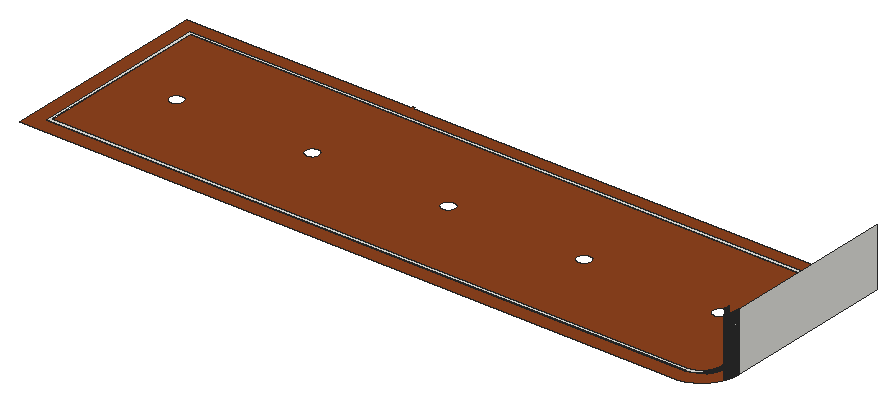
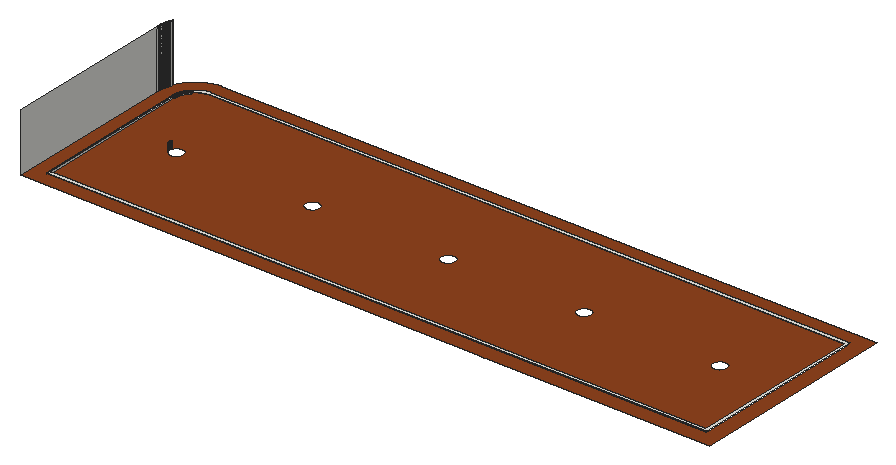
# SketchUp Ruby script. Lengths in inches.
U = 1.inch
M = Sketchup.active_model
def pt(a) = Geom::Point3d.new(a.map { |v| v * U })
def face(e, loops, mat)
  f = e.add_face(loops[0].map { |a| pt(a) })
  loops[1..].each { |l| e.add_face(l.map { |a| pt(a) }).erase! }
  f.material = f.back_material = mat if mat
  f
end
# faces: each face lists its corners as indices into pts; further lists are holes
def faces(e, pts, list, mat = nil) = list.each { |f| face(e, (f[0].is_a?(Array) ? f : [f]).map { |l| l.map { |i| pts[i] } }, mat) }
# xy, xz, yz: faces in a plane at the given z, y or x. An outline is a flat list of corners, or four numbers for a rectangle; further outlines are holes
def ring(l) = l.size == 4 ? [[l[0], l[1]], [l[2], l[1]], [l[2], l[3]], [l[0], l[3]]] : l.each_slice(2).to_a
def flat(e, list, mat, &to3) = list.each { |f| face(e, (f[0].is_a?(Array) ? f : [f]).map { |l| ring(l).map { |u, v| to3.(u, v) } }, mat) }
def xy(e, z, list, mat = nil) = flat(e, list, mat) { |x, y| [x, y, z] }
def xz(e, y, list, mat = nil) = flat(e, list, mat) { |x, z| [x, y, z] }
def yz(e, x, list, mat = nil) = flat(e, list, mat) { |y, z| [x, y, z] }
def lines(e, pts, list) = list.each { |a, b| e.add_line(pt(pts[a]), pt(pts[b])) }
# prism: a flat outline (further loops are holes) pulled along v
def prism(e, loops, v, mat = nil)
  f = face(e, loops, mat); d = Geom::Vector3d.new(v.map { |x| x * U })
  f.pushpull(f.normal.samedirection?(d) ? d.length : -d.length)
end
def box(e, o, s, mat = nil) = prism(e, [[o, [o[0] + s[0], o[1], o[2]], [o[0] + s[0], o[1] + s[1], o[2]], [o[0], o[1] + s[1], o[2]]]], [0, 0, s[2]], mat)
def at(x, y, z, deg = 0) = Geom::Transformation.translation(pt([x, y, z])) * Geom::Transformation.rotation(ORIGIN, Z_AXIS, deg.degrees)
def axes(o, x, y, z) = Geom::Transformation.new([*x, 0, *y, 0, *z, 0, *pt(o).to_a, 1])
def part(name) = M.definitions.add(name)
# library, detail: a bought-in or finely detailed component or shape, given as its bounding box
def library(name, o, s) = part(name).tap { |d| box(d.entities, o, s) }
def detail(e, o, s) = box(e.add_group.entities, o, s)
def put(e, d, t, mat = nil) = e.add_instance(d, t).tap { |i| i.material = mat if mat }
def group(e, t, mat = nil) = e.add_group.tap { |g| g.transformation = t; g.material = mat if mat }.entities
root = M.entities
M.materials.add("[Wood Fence]").color = [142, 67, 30]
xy(root,228,[[[99,214,99,300,191.5,300,191.5,300.5,192.5,300.5,192.5,300,383,300,383,229.12,382.99,228.93,382.98,228.73,382.96,228.35,382.86,227.4,382.74,226.64,382.7,226.46,382.58,225.89,382.53,225.71,382.48,225.52,382.43,225.34,382.38,225.15,382.33,224.97,382.27,224.79,382.21,224.6,382.09,224.24,382.02,224.0625,381.95,223.88,381.88,223.71,381.74,223.35,381.66,223.18,381.58,223,381.42,222.66,381.33,222.48,381.24,222.3125,381.15,222.14,381.0625,221.98,380.97,221.81,380.87,221.64,380.78,221.48,380.68,221.31,380.57,221.15,380.47,220.99,380.36,220.83,380.26,220.67,380.15,220.52,380.04,220.36,379.92,220.21,379.81,220.05,379.45,219.6,379.33,219.46,379.2,219.31,379.08,219.17,378.95,219.02,378.82,218.88,378.6875,218.74,378.56,218.61,378.15,218.2,378.01,218.07,377.86,217.94,377.72,217.8125,377.58,217.6875,377.43,217.56,376.98,217.2,376.83,217.09,376.68,216.97,376.52,216.86,376.37,216.75,376.05,216.53,375.89,216.43,375.73,216.32,375.57,216.22,375.4,216.125,375.24,216.03,375.07,215.93,374.91,215.84,374.4,215.57,374.22,215.49,374.05,215.41,373.88,215.32,373.7,215.25,373.53,215.17,373.35,215.1,373.17,215.02,372.99,214.95,372.82,214.89,372.64,214.82,372.45,214.76,371.91,214.58,371.72,214.53,371.54,214.48,371.35,214.43,371.17,214.38,370.98,214.34,370.8,214.29,370.61,214.25,370.42,214.22,370.23,214.18,369.85,214.12,369.67,214.09,369.48,214.0625,369.29,214.04,369.1,214.01,368.95,214],[105,220,368.62,220,368.6875,220.01,368.8,220.02,368.92,220.04,369.03,220.0625,369.15,220.08,369.27,220.1,369.38,220.13,369.5,220.15,369.61,220.18,369.73,220.21,369.84,220.23,369.95,220.27,370.07,220.3,370.29,220.36,370.41,220.4,370.52,220.4375,370.63,220.48,370.96,220.6,371.07,220.65,371.18,220.69,371.28,220.74,371.61,220.89,371.71,220.9375,371.82,220.99,371.92,221.05,372.02,221.1,372.23,221.22,372.63,221.46,372.73,221.53,372.83,221.59,372.92,221.66,373.02,221.73,373.11,221.8,373.21,221.87,373.39,222.01,373.49,222.09,373.58,222.16,373.76,222.32,373.84,222.39,374.02,222.55,374.1,222.64,374.18,222.72,374.27,222.8,374.35,222.89,374.43,222.97,374.67,223.24,374.74,223.32,374.82,223.42,374.89,223.51,374.97,223.6,375.04,223.69,375.11,223.79,375.18,223.88,375.25,223.98,375.3125,224.07,375.38,224.17,375.44,224.27,375.51,224.37,375.75,224.77,375.81,224.875,375.86,224.98,375.92,225.08,375.97,225.1875,376.03,225.29,376.08,225.4,376.125,225.51,376.18,225.61,376.22,225.72,376.27,225.83,376.3125,225.9375,376.36,226.05,376.4,226.16,376.4375,226.27,376.48,226.38,376.51,226.49,376.55,226.6,376.59,226.72,376.68,227.05,376.71,227.17,376.74,227.28,376.77,227.4,376.79,227.51,376.82,227.63,376.84,227.74,376.88,227.98,376.9,228.09,376.91,228.21,376.93,228.33,376.94,228.44,376.96,228.68,376.97,228.79,376.99,229.03,376.99,229.15,377,229.26,377,294,105,294]],[[106,221,106,293,376,293,376,229.29,375.99,229.18,375.99,229.08,375.98,228.97,375.98,228.87,375.97,228.76,375.96,228.66,375.95,228.55,375.94,228.45,375.92,228.34,375.91,228.24,375.89,228.14,375.875,228.03,375.85,227.93,375.83,227.82,375.8125,227.72,375.79,227.62,375.77,227.51,375.74,227.41,375.72,227.31,375.6875,227.21,375.66,227.11,375.6,226.91,375.57,226.8,375.53,226.71,375.5,226.61,375.34,226.21,375.3,226.12,375.22,225.92,375.17,225.83,375.13,225.73,375.08,225.64,375.03,225.54,374.88,225.27,374.83,225.17,374.78,225.08,374.66,224.9,374.61,224.82,374.43,224.55,374.37,224.47,374.31,224.38,374.24,224.3,374.18,224.22,374.11,224.13,374.05,224.05,373.7,223.65,373.625,223.58,373.55,223.5,373.33,223.28,372.85,222.86,372.77,222.8,372.6875,222.73,372.6,222.67,372.52,222.6,372.43,222.54,372.35,222.48,372.17,222.36,372.09,222.3,372,222.25,371.91,222.19,371.82,222.14,371.73,222.08,371.64,222.03,371.54,221.98,371.36,221.88,371.26,221.83,371.17,221.79,371.07,221.74,370.98,221.7,370.88,221.65,370.78,221.61,370.6875,221.57,370.59,221.53,370.49,221.49,370.39,221.46,370.19,221.38,369.59,221.2,369.49,221.18,369.38,221.15,369.18,221.11,369.07,221.09,368.87,221.05,368.76,221.03,368.66,221.01,368.56,221],[184.84,254,185.16,254,185.24,254.01,185.3125,254.02,185.39,254.03,185.55,254.05,185.625,254.07,185.7,254.08,185.78,254.1,185.85,254.125,185.93,254.15,186,254.17,186.08,254.2,186.29,254.29,186.36,254.33,186.43,254.36,186.57,254.44,186.63,254.48,186.7,254.53,186.76,254.57,186.83,254.62,187.07,254.82,187.12,254.88,187.18,254.93,187.38,255.17,187.43,255.24,187.47,255.3,187.52,255.37,187.56,255.43,187.64,255.57,187.67,255.64,187.71,255.71,187.8,255.92,187.83,256,187.85,256.07,187.875,256.15,187.9,256.22,187.92,256.3,187.93,256.375,187.95,256.45,187.97,256.61,187.98,256.6875,187.99,256.76,188,256.84,188,257.16,187.99,257.24,187.98,257.3125,187.97,257.39,187.95,257.55,187.93,257.625,187.92,257.7,187.9,257.78,187.875,257.85,187.85,257.93,187.83,258,187.8,258.08,187.71,258.29,187.67,258.36,187.64,258.43,187.56,258.57,187.52,258.63,187.47,258.7,187.43,258.76,187.38,258.83,187.18,259.07,187.12,259.12,187.07,259.18,186.83,259.38,186.76,259.43,186.7,259.47,186.63,259.52,186.57,259.56,186.43,259.64,186.36,259.67,186.29,259.71,186.08,259.8,186,259.83,185.93,259.85,185.85,259.875,185.78,259.9,185.7,259.92,185.625,259.93,185.55,259.95,185.39,259.97,185.3125,259.98,185.24,259.99,185.16,260,184.84,260,184.76,259.99,184.6875,259.98,184.61,259.97,184.45,259.95,184.375,259.93,184.3,259.92,184.22,259.9,184.15,259.875,184.07,259.85,184,259.83,183.92,259.8,183.71,259.71,183.64,259.67,183.57,259.64,183.43,259.56,183.37,259.52,183.3,259.47,183.24,259.43,183.17,259.38,182.93,259.18,182.88,259.12,182.82,259.07,182.62,258.83,182.57,258.76,182.53,258.7,182.48,258.63,182.44,258.57,182.36,258.43,182.33,258.36,182.29,258.29,182.2,258.08,182.17,258,182.15,257.93,182.125,257.85,182.1,257.78,182.08,257.7,182.07,257.625,182.05,257.55,182.03,257.39,182.02,257.3125,182.01,257.24,182,257.16,182,256.84,182.01,256.76,182.02,256.6875,182.03,256.61,182.05,256.45,182.07,256.375,182.08,256.3,182.1,256.22,182.125,256.15,182.15,256.07,182.17,256,182.2,255.92,182.29,255.71,182.33,255.64,182.36,255.57,182.44,255.43,182.48,255.37,182.53,255.3,182.57,255.24,182.62,255.17,182.82,254.93,182.88,254.88,182.93,254.82,183.17,254.62,183.24,254.57,183.3,254.53,183.37,254.48,183.43,254.44,183.57,254.36,183.64,254.33,183.71,254.29,183.92,254.2,184,254.17,184.07,254.15,184.15,254.125,184.22,254.1,184.3,254.08,184.375,254.07,184.45,254.05,184.61,254.03,184.6875,254.02,184.76,254.01],[240.84,254,241.16,254,241.24,254.01,241.3125,254.02,241.39,254.03,241.55,254.05,241.625,254.07,241.7,254.08,241.78,254.1,241.85,254.125,241.93,254.15,242,254.17,242.08,254.2,242.29,254.29,242.36,254.33,242.43,254.36,242.57,254.44,242.63,254.48,242.7,254.53,242.76,254.57,242.83,254.62,243.07,254.82,243.12,254.88,243.18,254.93,243.38,255.17,243.43,255.24,243.47,255.3,243.52,255.37,243.56,255.43,243.64,255.57,243.67,255.64,243.71,255.71,243.8,255.92,243.83,256,243.85,256.07,243.875,256.15,243.9,256.22,243.92,256.3,243.93,256.375,243.95,256.45,243.97,256.61,243.98,256.6875,243.99,256.76,244,256.84,244,257.16,243.99,257.24,243.98,257.3125,243.97,257.39,243.95,257.55,243.93,257.625,243.92,257.7,243.9,257.78,243.875,257.85,243.85,257.93,243.83,258,243.8,258.08,243.71,258.29,243.67,258.36,243.64,258.43,243.56,258.57,243.52,258.63,243.47,258.7,243.43,258.76,243.38,258.83,243.18,259.07,243.12,259.12,243.07,259.18,242.83,259.38,242.76,259.43,242.7,259.47,242.63,259.52,242.57,259.56,242.43,259.64,242.36,259.67,242.29,259.71,242.08,259.8,242,259.83,241.93,259.85,241.85,259.875,241.78,259.9,241.7,259.92,241.625,259.93,241.55,259.95,241.39,259.97,241.3125,259.98,241.24,259.99,241.16,260,240.84,260,240.76,259.99,240.6875,259.98,240.61,259.97,240.45,259.95,240.375,259.93,240.3,259.92,240.22,259.9,240.15,259.875,240.07,259.85,240,259.83,239.92,259.8,239.71,259.71,239.64,259.67,239.57,259.64,239.43,259.56,239.37,259.52,239.3,259.47,239.24,259.43,239.17,259.38,238.93,259.18,238.88,259.12,238.82,259.07,238.62,258.83,238.57,258.76,238.53,258.7,238.48,258.63,238.44,258.57,238.36,258.43,238.33,258.36,238.29,258.29,238.2,258.08,238.17,258,238.15,257.93,238.125,257.85,238.1,257.78,238.08,257.7,238.07,257.625,238.05,257.55,238.03,257.39,238.02,257.3125,238.01,257.24,238,257.16,238,256.84,238.01,256.76,238.02,256.6875,238.03,256.61,238.05,256.45,238.07,256.375,238.08,256.3,238.1,256.22,238.125,256.15,238.15,256.07,238.17,256,238.2,255.92,238.29,255.71,238.33,255.64,238.36,255.57,238.44,255.43,238.48,255.37,238.53,255.3,238.57,255.24,238.62,255.17,238.82,254.93,238.88,254.88,238.93,254.82,239.17,254.62,239.24,254.57,239.3,254.53,239.37,254.48,239.43,254.44,239.57,254.36,239.64,254.33,239.71,254.29,239.92,254.2,240,254.17,240.07,254.15,240.15,254.125,240.22,254.1,240.3,254.08,240.375,254.07,240.45,254.05,240.61,254.03,240.6875,254.02,240.76,254.01],[128.84,254,129.16,254,129.24,254.01,129.3125,254.02,129.39,254.03,129.55,254.05,129.625,254.07,129.7,254.08,129.78,254.1,129.85,254.125,129.93,254.15,130,254.17,130.08,254.2,130.29,254.29,130.36,254.33,130.43,254.36,130.57,254.44,130.63,254.48,130.7,254.53,130.76,254.57,130.83,254.62,131.07,254.82,131.12,254.88,131.18,254.93,131.38,255.17,131.43,255.24,131.47,255.3,131.52,255.37,131.56,255.43,131.64,255.57,131.67,255.64,131.71,255.71,131.8,255.92,131.83,256,131.85,256.07,131.875,256.15,131.9,256.22,131.92,256.3,131.93,256.375,131.95,256.45,131.97,256.61,131.98,256.6875,131.99,256.76,132,256.84,132,257.16,131.99,257.24,131.98,257.3125,131.97,257.39,131.95,257.55,131.93,257.625,131.92,257.7,131.9,257.78,131.875,257.85,131.85,257.93,131.83,258,131.8,258.08,131.71,258.29,131.67,258.36,131.64,258.43,131.56,258.57,131.52,258.63,131.47,258.7,131.43,258.76,131.38,258.83,131.18,259.07,131.12,259.12,131.07,259.18,130.83,259.38,130.76,259.43,130.7,259.47,130.63,259.52,130.57,259.56,130.43,259.64,130.36,259.67,130.29,259.71,130.08,259.8,130,259.83,129.93,259.85,129.85,259.875,129.78,259.9,129.7,259.92,129.625,259.93,129.55,259.95,129.39,259.97,129.3125,259.98,129.24,259.99,129.16,260,128.84,260,128.76,259.99,128.6875,259.98,128.61,259.97,128.45,259.95,128.375,259.93,128.3,259.92,128.22,259.9,128.15,259.875,128.07,259.85,128,259.83,127.92,259.8,127.71,259.71,127.64,259.67,127.57,259.64,127.43,259.56,127.37,259.52,127.3,259.47,127.24,259.43,127.17,259.38,126.93,259.18,126.88,259.12,126.82,259.07,126.62,258.83,126.57,258.76,126.53,258.7,126.48,258.63,126.44,258.57,126.36,258.43,126.33,258.36,126.29,258.29,126.2,258.08,126.17,258,126.15,257.93,126.125,257.85,126.1,257.78,126.08,257.7,126.07,257.625,126.05,257.55,126.03,257.39,126.02,257.3125,126.01,257.24,126,257.16,126,256.84,126.01,256.76,126.02,256.6875,126.03,256.61,126.05,256.45,126.07,256.375,126.08,256.3,126.1,256.22,126.125,256.15,126.15,256.07,126.17,256,126.2,255.92,126.29,255.71,126.33,255.64,126.36,255.57,126.44,255.43,126.48,255.37,126.53,255.3,126.57,255.24,126.62,255.17,126.82,254.93,126.88,254.88,126.93,254.82,127.17,254.62,127.24,254.57,127.3,254.53,127.37,254.48,127.43,254.44,127.57,254.36,127.64,254.33,127.71,254.29,127.92,254.2,128,254.17,128.07,254.15,128.15,254.125,128.22,254.1,128.3,254.08,128.375,254.07,128.45,254.05,128.61,254.03,128.6875,254.02,128.76,254.01],[296.84,254,297.16,254,297.24,254.01,297.3125,254.02,297.39,254.03,297.55,254.05,297.625,254.07,297.7,254.08,297.78,254.1,297.85,254.125,297.93,254.15,298,254.17,298.08,254.2,298.29,254.29,298.36,254.33,298.43,254.36,298.57,254.44,298.63,254.48,298.7,254.53,298.76,254.57,298.83,254.62,299.07,254.82,299.12,254.88,299.18,254.93,299.38,255.17,299.43,255.24,299.47,255.3,299.52,255.37,299.56,255.43,299.64,255.57,299.67,255.64,299.71,255.71,299.8,255.92,299.83,256,299.85,256.07,299.875,256.15,299.9,256.22,299.92,256.3,299.93,256.375,299.95,256.45,299.97,256.61,299.98,256.6875,299.99,256.76,300,256.84,300,257.16,299.99,257.24,299.98,257.3125,299.97,257.39,299.95,257.55,299.93,257.625,299.92,257.7,299.9,257.78,299.875,257.85,299.85,257.93,299.83,258,299.8,258.08,299.71,258.29,299.67,258.36,299.64,258.43,299.56,258.57,299.52,258.63,299.47,258.7,299.43,258.76,299.38,258.83,299.18,259.07,299.12,259.12,299.07,259.18,298.83,259.38,298.76,259.43,298.7,259.47,298.63,259.52,298.57,259.56,298.43,259.64,298.36,259.67,298.29,259.71,298.08,259.8,298,259.83,297.93,259.85,297.85,259.875,297.78,259.9,297.7,259.92,297.625,259.93,297.55,259.95,297.39,259.97,297.3125,259.98,297.24,259.99,297.16,260,296.84,260,296.76,259.99,296.6875,259.98,296.61,259.97,296.45,259.95,296.375,259.93,296.3,259.92,296.22,259.9,296.15,259.875,296.07,259.85,296,259.83,295.92,259.8,295.71,259.71,295.64,259.67,295.57,259.64,295.43,259.56,295.37,259.52,295.3,259.47,295.24,259.43,295.17,259.38,294.93,259.18,294.88,259.12,294.82,259.07,294.62,258.83,294.57,258.76,294.53,258.7,294.48,258.63,294.44,258.57,294.36,258.43,294.33,258.36,294.29,258.29,294.2,258.08,294.17,258,294.15,257.93,294.125,257.85,294.1,257.78,294.08,257.7,294.07,257.625,294.05,257.55,294.03,257.39,294.02,257.3125,294.01,257.24,294,257.16,294,256.84,294.01,256.76,294.02,256.6875,294.03,256.61,294.05,256.45,294.07,256.375,294.08,256.3,294.1,256.22,294.125,256.15,294.15,256.07,294.17,256,294.2,255.92,294.29,255.71,294.33,255.64,294.36,255.57,294.44,255.43,294.48,255.37,294.53,255.3,294.57,255.24,294.62,255.17,294.82,254.93,294.88,254.88,294.93,254.82,295.17,254.62,295.24,254.57,295.3,254.53,295.37,254.48,295.43,254.44,295.57,254.36,295.64,254.33,295.71,254.29,295.92,254.2,296,254.17,296.07,254.15,296.15,254.125,296.22,254.1,296.3,254.08,296.375,254.07,296.45,254.05,296.61,254.03,296.6875,254.02,296.76,254.01],[352.84,254,353.16,254,353.24,254.01,353.3125,254.02,353.39,254.03,353.55,254.05,353.625,254.07,353.7,254.08,353.78,254.1,353.85,254.125,353.93,254.15,354,254.17,354.08,254.2,354.29,254.29,354.36,254.33,354.43,254.36,354.57,254.44,354.63,254.48,354.7,254.53,354.76,254.57,354.83,254.62,355.07,254.82,355.12,254.88,355.18,254.93,355.38,255.17,355.43,255.24,355.47,255.3,355.52,255.37,355.56,255.43,355.64,255.57,355.67,255.64,355.71,255.71,355.8,255.92,355.83,256,355.85,256.07,355.875,256.15,355.9,256.22,355.92,256.3,355.93,256.375,355.95,256.45,355.97,256.61,355.98,256.6875,355.99,256.76,356,256.84,356,257.16,355.99,257.24,355.98,257.3125,355.97,257.39,355.95,257.55,355.93,257.625,355.92,257.7,355.9,257.78,355.875,257.85,355.85,257.93,355.83,258,355.8,258.08,355.71,258.29,355.67,258.36,355.64,258.43,355.56,258.57,355.52,258.63,355.47,258.7,355.43,258.76,355.38,258.83,355.18,259.07,355.12,259.12,355.07,259.18,354.83,259.38,354.76,259.43,354.7,259.47,354.63,259.52,354.57,259.56,354.43,259.64,354.36,259.67,354.29,259.71,354.08,259.8,354,259.83,353.93,259.85,353.85,259.875,353.78,259.9,353.7,259.92,353.625,259.93,353.55,259.95,353.39,259.97,353.3125,259.98,353.24,259.99,353.16,260,352.84,260,352.76,259.99,352.6875,259.98,352.61,259.97,352.45,259.95,352.375,259.93,352.3,259.92,352.22,259.9,352.15,259.875,352.07,259.85,352,259.83,351.92,259.8,351.71,259.71,351.64,259.67,351.57,259.64,351.43,259.56,351.37,259.52,351.3,259.47,351.24,259.43,351.17,259.38,350.93,259.18,350.88,259.12,350.82,259.07,350.62,258.83,350.57,258.76,350.53,258.7,350.48,258.63,350.44,258.57,350.36,258.43,350.33,258.36,350.29,258.29,350.2,258.08,350.17,258,350.15,257.93,350.125,257.85,350.1,257.78,350.08,257.7,350.07,257.625,350.05,257.55,350.03,257.39,350.02,257.3125,350.01,257.24,350,257.16,350,256.84,350.01,256.76,350.02,256.6875,350.03,256.61,350.05,256.45,350.07,256.375,350.08,256.3,350.1,256.22,350.125,256.15,350.15,256.07,350.17,256,350.2,255.92,350.29,255.71,350.33,255.64,350.36,255.57,350.44,255.43,350.48,255.37,350.53,255.3,350.57,255.24,350.62,255.17,350.82,254.93,350.88,254.88,350.93,254.82,351.17,254.62,351.24,254.57,351.3,254.53,351.37,254.48,351.43,254.44,351.57,254.36,351.64,254.33,351.71,254.29,351.92,254.2,352,254.17,352.07,254.15,352.15,254.125,352.22,254.1,352.3,254.08,352.375,254.07,352.45,254.05,352.61,254.03,352.6875,254.02,352.76,254.01]]],"[Wood Fence]")
xy(root,228.5,[[[105,220,105,294,377,294,377,229.26,376.99,229.15,376.99,229.03,376.97,228.79,376.96,228.68,376.94,228.44,376.93,228.33,376.91,228.21,376.9,228.09,376.88,227.98,376.84,227.74,376.82,227.63,376.79,227.51,376.77,227.4,376.74,227.28,376.71,227.17,376.68,227.05,376.59,226.72,376.55,226.6,376.51,226.49,376.48,226.38,376.4375,226.27,376.4,226.16,376.36,226.05,376.3125,225.9375,376.27,225.83,376.22,225.72,376.18,225.61,376.125,225.51,376.08,225.4,376.03,225.29,375.97,225.1875,375.92,225.08,375.86,224.98,375.81,224.875,375.75,224.77,375.51,224.37,375.44,224.27,375.38,224.17,375.3125,224.07,375.25,223.98,375.18,223.88,375.11,223.79,375.04,223.69,374.97,223.6,374.89,223.51,374.82,223.42,374.74,223.32,374.67,223.24,374.43,222.97,374.35,222.89,374.27,222.8,374.18,222.72,374.1,222.64,374.02,222.55,373.84,222.39,373.76,222.32,373.58,222.16,373.49,222.09,373.39,222.01,373.21,221.87,373.11,221.8,373.02,221.73,372.92,221.66,372.83,221.59,372.73,221.53,372.63,221.46,372.23,221.22,372.02,221.1,371.92,221.05,371.82,220.99,371.71,220.9375,371.61,220.89,371.28,220.74,371.18,220.69,371.07,220.65,370.96,220.6,370.63,220.48,370.52,220.4375,370.41,220.4,370.29,220.36,370.07,220.3,369.95,220.27,369.84,220.23,369.73,220.21,369.61,220.18,369.5,220.15,369.38,220.13,369.27,220.1,369.15,220.08,369.03,220.0625,368.92,220.04,368.8,220.02,368.6875,220.01,368.62,220],[106,221,368.56,221,368.66,221.01,368.76,221.03,368.87,221.05,369.07,221.09,369.18,221.11,369.38,221.15,369.49,221.18,369.59,221.2,370.19,221.38,370.39,221.46,370.49,221.49,370.59,221.53,370.6875,221.57,370.78,221.61,370.88,221.65,370.98,221.7,371.07,221.74,371.17,221.79,371.26,221.83,371.36,221.88,371.54,221.98,371.64,222.03,371.73,222.08,371.82,222.14,371.91,222.19,372,222.25,372.09,222.3,372.17,222.36,372.35,222.48,372.43,222.54,372.52,222.6,372.6,222.67,372.6875,222.73,372.77,222.8,372.85,222.86,373.33,223.28,373.55,223.5,373.625,223.58,373.7,223.65,374.05,224.05,374.11,224.13,374.18,224.22,374.24,224.3,374.31,224.38,374.37,224.47,374.43,224.55,374.61,224.82,374.66,224.9,374.78,225.08,374.83,225.17,374.88,225.27,375.03,225.54,375.08,225.64,375.13,225.73,375.17,225.83,375.22,225.92,375.3,226.12,375.34,226.21,375.5,226.61,375.53,226.71,375.57,226.8,375.6,226.91,375.66,227.11,375.6875,227.21,375.72,227.31,375.74,227.41,375.77,227.51,375.79,227.62,375.8125,227.72,375.83,227.82,375.85,227.93,375.875,228.03,375.89,228.14,375.91,228.24,375.92,228.34,375.94,228.45,375.95,228.55,375.96,228.66,375.97,228.76,375.98,228.87,375.98,228.97,375.99,229.08,375.99,229.18,376,229.29,376,293,106,293]]])
yz(root,356,[[256.84,228,256.92,231],[256.92,228,257,231],[257,228,257.08,231],[257.08,228,257.16,231]])
yz(root,375.98,[[228.87,228,228.97,228.5]])
yz(root,375.99,[[229.08,228,229.18,228.5]])
yz(root,376,[[229.29,228,229.39,228.5],[229.39,228,229.52,228.5],[229.52,228,293,228.5]])
yz(root,376.99,[[229.03,228,229.15,228.5]])
yz(root,377,[[229.26,228,229.38,228.5],[229.38,228,229.52,228.5],[229.52,228,294,228.5]])
yz(root,383,[[229.12,228,229.31,252],[229.31,228,229.5,252],[229.5,228,300,252]])
p = [[373.25,223.21,228],[373.33,223.28,228],[373.33,223.28,228.5],[373.25,223.21,228.5],[374.74,223.32,228],[374.67,223.24,228],
  [374.67,223.24,228.5],[374.74,223.32,228.5],[381.66,223.18,228],[381.74,223.35,228],[381.74,223.35,252],[381.66,223.18,252],
  [373.4,223.35,228],[373.4,223.35,228.5],[374.82,223.42,228],[374.82,223.42,228.5],[373.48,223.43,228],[373.48,223.43,228.5],
  [373.55,223.5,228],[373.55,223.5,228.5],[374.89,223.51,228],[374.89,223.51,228.5],[381.81,223.53,228],[381.81,223.53,252],
  [373.625,223.58,228],[373.625,223.58,228.5],[374.97,223.6,228],[374.97,223.6,228.5],[381.88,223.71,228],[381.88,223.71,252],
  [373.7,223.65,228],[373.7,223.65,228.5],[375.04,223.69,228],[375.04,223.69,228.5],[373.77,223.73,228],[373.77,223.73,228.5],
  [373.84,223.81,228],[373.84,223.81,228.5],[375.11,223.79,228],[375.11,223.79,228.5],[381.95,223.88,228],[381.95,223.88,252],
  [373.91,223.89,228],[373.91,223.89,228.5],[375.18,223.88,228],[375.18,223.88,228.5],[373.98,223.97,228],[373.98,223.97,228.5],
  [375.25,223.98,228],[375.25,223.98,228.5],[382.02,224.0625,228],[382.02,224.0625,252],[374.05,224.05,228],[374.05,224.05,228.5],
  [375.3125,224.07,228],[375.3125,224.07,228.5],[374.11,224.13,228],[374.11,224.13,228.5],[374.18,224.22,228],[374.18,224.22,228.5],
  [375.38,224.17,228],[375.38,224.17,228.5],[382.09,224.24,228],[382.09,224.24,252],[374.24,224.3,228],[374.24,224.3,228.5],
  [375.44,224.27,228],[375.44,224.27,228.5],[382.15,224.42,228],[382.15,224.42,252],[374.31,224.38,228],[374.31,224.38,228.5],
  [375.51,224.37,228],[375.51,224.37,228.5],[374.37,224.47,228],[374.37,224.47,228.5],[375.57,224.47,228],[375.57,224.47,228.5],
  [382.21,224.6,228],[382.21,224.6,252],[374.43,224.55,228],[374.43,224.55,228.5],[375.63,224.57,228],[375.63,224.57,228.5],
  [374.49,224.64,228],[374.49,224.64,228.5],[374.55,224.73,228],[374.55,224.73,228.5],[375.69,224.67,228],[375.69,224.67,228.5],
  [382.27,224.79,228],[382.27,224.79,252],[374.61,224.82,228],[374.61,224.82,228.5],[375.75,224.77,228],[375.75,224.77,228.5],
  [374.66,224.9,228],[374.66,224.9,228.5],[375.81,224.875,228],[375.81,224.875,228.5],[382.33,224.97,228],[382.33,224.97,252],
  [374.72,224.99,228],[374.72,224.99,228.5],[375.86,224.98,228],[375.86,224.98,228.5],[374.78,225.08,228],[374.78,225.08,228.5],
  [375.92,225.08,228],[375.92,225.08,228.5],[382.38,225.15,228],[382.38,225.15,252],[374.83,225.17,228],[374.83,225.17,228.5],
  [375.97,225.1875,228],[375.97,225.1875,228.5],[374.88,225.27,228],[374.88,225.27,228.5],[376.03,225.29,228],[376.03,225.29,228.5],
  [382.43,225.34,228],[382.43,225.34,252],[374.93,225.36,228],[374.93,225.36,228.5],[376.08,225.4,228],[376.08,225.4,228.5],
  [382.48,225.52,228],[382.48,225.52,252],[374.98,225.45,228],[374.98,225.45,228.5],[376.125,225.51,228],[376.125,225.51,228.5],
  [375.03,225.54,228],[375.03,225.54,228.5],[375.08,225.64,228],[375.08,225.64,228.5],[376.18,225.61,228],[376.18,225.61,228.5],
  [382.53,225.71,228],[382.53,225.71,252],[375.13,225.73,228],[375.13,225.73,228.5],[376.22,225.72,228],[376.22,225.72,228.5],
  [375.17,225.83,228],[375.17,225.83,228.5],[376.27,225.83,228],[376.27,225.83,228.5],[382.58,225.89,228],[382.58,225.89,252],
  [375.22,225.92,228],[375.22,225.92,228.5],[376.3125,225.9375,228],[376.3125,225.9375,228.5],[375.26,226.02,228],[375.26,226.02,228.5],
  [376.36,226.05,228],[376.36,226.05,228.5],[382.62,226.08,228],[382.62,226.08,252],[375.3,226.12,228],[375.3,226.12,228.5],
  [376.4,226.16,228],[376.4,226.16,228.5],[375.34,226.21,228],[375.34,226.21,228.5],[382.66,226.27,228],[382.66,226.27,252],
  [375.38,226.31,228],[375.38,226.31,228.5],[376.4375,226.27,228],[376.4375,226.27,228.5],[375.42,226.41,228],[375.42,226.41,228.5],
  [376.48,226.38,228],[376.48,226.38,228.5],[382.7,226.46,228],[382.7,226.46,252],[375.46,226.51,228],[375.46,226.51,228.5],
  [376.51,226.49,228],[376.51,226.49,228.5],[375.5,226.61,228],[375.5,226.61,228.5],[376.55,226.6,228],[376.55,226.6,228.5],
  [382.74,226.64,228],[382.74,226.64,252],[375.53,226.71,228],[375.53,226.71,228.5],[376.59,226.72,228],[376.59,226.72,228.5],
  [382.77,226.83,228],[382.77,226.83,252],[375.57,226.8,228],[375.57,226.8,228.5],[376.62,226.83,228],[376.62,226.83,228.5],
  [375.6,226.91,228],[375.6,226.91,228.5],[376.65,226.94,228],[376.65,226.94,228.5],[382.8,227.02,228],[382.8,227.02,252],
  [375.63,227.01,228],[375.63,227.01,228.5],[376.68,227.05,228],[376.68,227.05,228.5],[375.66,227.11,228],[375.66,227.11,228.5],
  [382.83,227.21,228],[382.83,227.21,252],[375.6875,227.21,228],[375.6875,227.21,228.5],[376.71,227.17,228],[376.71,227.17,228.5],
  [375.72,227.31,228],[375.72,227.31,228.5],[376.74,227.28,228],[376.74,227.28,228.5],[382.86,227.4,228],[382.86,227.4,252],
  [375.74,227.41,228],[375.74,227.41,228.5],[376.77,227.4,228],[376.77,227.4,228.5],[375.77,227.51,228],[375.77,227.51,228.5],
  [376.79,227.51,228],[376.79,227.51,228.5],[382.88,227.59,228],[382.88,227.59,252],[375.79,227.62,228],[375.79,227.62,228.5],
  [376.82,227.63,228],[376.82,227.63,228.5],[375.8125,227.72,228],[375.8125,227.72,228.5],[376.84,227.74,228],[376.84,227.74,228.5],
  [382.9,227.78,228],[382.9,227.78,252],[375.83,227.82,228],[375.83,227.82,228.5],[376.86,227.86,228],[376.86,227.86,228.5],
  [375.85,227.93,228],[375.85,227.93,228.5],[382.92,227.97,228],[382.92,227.97,252],[375.875,228.03,228],[375.875,228.03,228.5],
  [376.88,227.98,228],[376.88,227.98,228.5],[375.89,228.14,228],[375.89,228.14,228.5],[376.9,228.09,228],[376.9,228.09,228.5],
  [382.94,228.16,228],[382.94,228.16,252],[375.91,228.24,228],[375.91,228.24,228.5],[376.91,228.21,228],[376.91,228.21,228.5],
  [375.92,228.34,228],[375.92,228.34,228.5],[376.93,228.33,228],[376.93,228.33,228.5],[382.96,228.35,228],[382.96,228.35,252],
  [375.94,228.45,228],[375.94,228.45,228.5],[376.94,228.44,228],[376.94,228.44,228.5],[375.95,228.55,228],[375.95,228.55,228.5],
  [376.95,228.56,228],[376.95,228.56,228.5],[382.97,228.54,228],[382.97,228.54,252],[382.98,228.73,228],[382.98,228.73,252],
  [375.96,228.66,228],[375.96,228.66,228.5],[376.96,228.68,228],[376.96,228.68,228.5],[375.97,228.76,228],[375.97,228.76,228.5],
  [376.97,228.79,228],[376.97,228.79,228.5],[382.99,228.93,228],[382.99,228.93,252],[375.98,228.87,228],[375.98,228.87,228.5],
  [376.98,228.91,228],[376.98,228.91,228.5],[376.99,229.03,228],[376.99,229.03,228.5],[383,229.12,228],[383,229.12,252],
  [375.98,228.97,228],[375.99,229.08,228],[375.99,229.08,228.5],[375.98,228.97,228.5],[377,229.26,228],[376.99,229.15,228],
  [376.99,229.15,228.5],[377,229.26,228.5],[375.99,229.18,228],[376,229.29,228],[376,229.29,228.5],[375.99,229.18,228.5],
  [355.77,255.85,228],[355.74,255.78,228],[355.74,255.78,231],[355.77,255.85,231],[355.8,255.92,228],[355.8,255.92,231],
  [355.83,256,228],[355.83,256,231],[355.85,256.07,228],[355.85,256.07,231],[355.875,256.15,228],[355.875,256.15,231],
  [355.9,256.22,228],[355.9,256.22,231],[355.92,256.3,228],[355.92,256.3,231],[355.93,256.375,228],[355.93,256.375,231],
  [355.95,256.45,228],[355.95,256.45,231],[355.96,256.53,228],[355.96,256.53,231],[355.97,256.61,228],[355.97,256.61,231],
  [355.98,256.6875,228],[355.98,256.6875,231],[355.99,256.76,228],[355.99,256.76,231],[356,256.84,228],[356,256.84,231],
  [355.99,257.24,228],[356,257.16,228],[356,257.16,231],[355.99,257.24,231],[355.98,257.3125,228],[355.98,257.3125,231],
  [355.97,257.39,228],[355.97,257.39,231],[355.96,257.47,228],[355.96,257.47,231],[355.95,257.55,228],[355.95,257.55,231],
  [355.93,257.625,228],[355.93,257.625,231],[355.92,257.7,228],[355.92,257.7,231],[355.9,257.78,228],[355.9,257.78,231],
  [355.875,257.85,228],[355.875,257.85,231],[355.83,258,228],[355.85,257.93,228],[355.85,257.93,231],[355.83,258,231],
  [355.8,258.08,228],[355.8,258.08,231],[355.74,258.22,228],[355.77,258.15,228],[355.77,258.15,231],[355.74,258.22,231]]
faces(root,p,[[0,1,2,3],[4,5,6,7],[8,9,10,11],[1,12,13,2],[14,4,7,15],[12,16,17,13],[16,18,19,17],[20,14,15,21],
  [9,22,23,10],[18,24,25,19],[26,20,21,27],[22,28,29,23],[24,30,31,25],[32,26,27,33],[30,34,35,31],[34,36,37,35],
  [38,32,33,39],[28,40,41,29],[36,42,43,37],[44,38,39,45],[42,46,47,43],[48,44,45,49],[40,50,51,41],[46,52,53,47],
  [54,48,49,55],[52,56,57,53],[56,58,59,57],[60,54,55,61],[50,62,63,51],[58,64,65,59],[66,60,61,67],[62,68,69,63],
  [64,70,71,65],[72,66,67,73],[70,74,75,71],[76,72,73,77],[68,78,79,69],[74,80,81,75],[82,76,77,83],[80,84,85,81],
  [84,86,87,85],[88,82,83,89],[78,90,91,79],[86,92,93,87],[94,88,89,95],[92,96,97,93],[98,94,95,99],[90,100,101,91],
  [96,102,103,97],[104,98,99,105],[102,106,107,103],[108,104,105,109],[100,110,111,101],[106,112,113,107],[114,108,109,115],[112,116,117,113],
  [118,114,115,119],[110,120,121,111],[116,122,123,117],[124,118,119,125],[120,126,127,121],[122,128,129,123],[130,124,125,131],[128,132,133,129],
  [132,134,135,133],[136,130,131,137],[126,138,139,127],[134,140,141,135],[142,136,137,143],[140,144,145,141],[146,142,143,147],[138,148,149,139],
  [144,150,151,145],[152,146,147,153],[150,154,155,151],[156,152,153,157],[148,158,159,149],[154,160,161,155],[162,156,157,163],[160,164,165,161],
  [158,166,167,159],[164,168,169,165],[170,162,163,171],[168,172,173,169],[174,170,171,175],[166,176,177,167],[172,178,179,173],[180,174,175,181],
  [178,182,183,179],[184,180,181,185],[176,186,187,177],[182,188,189,183],[190,184,185,191],[186,192,193,187],[188,194,195,189],[196,190,191,197],
  [194,198,199,195],[200,196,197,201],[192,202,203,193],[198,204,205,199],[206,200,201,207],[204,208,209,205],[202,210,211,203],[208,212,213,209],
  [214,206,207,215],[212,216,217,213],[218,214,215,219],[210,220,221,211],[216,222,223,217],[224,218,219,225],[222,226,227,223],[228,224,225,229],
  [220,230,231,221],[226,232,233,227],[234,228,229,235],[232,236,237,233],[238,234,235,239],[230,240,241,231],[236,242,243,237],[244,238,239,245],
  [242,246,247,243],[240,248,249,241],[246,250,251,247],[252,244,245,253],[250,254,255,251],[256,252,253,257],[248,258,259,249],[254,260,261,255],
  [262,256,257,263],[260,264,265,261],[266,262,263,267],[258,268,269,259],[264,270,271,265],[272,266,267,273],[270,274,275,271],[276,272,273,277],
  [268,278,279,269],[278,280,281,279],[274,282,283,275],[284,276,277,285],[282,286,287,283],[288,284,285,289],[280,290,291,281],[286,292,293,287],
  [294,288,289,295],[296,294,295,297],[290,298,299,291],[300,301,302,303],[304,305,306,307],[308,309,310,311],[312,313,314,315],[316,312,315,317],
  [318,316,317,319],[320,318,319,321],[322,320,321,323],[324,322,323,325],[326,324,325,327],[328,326,327,329],[330,328,329,331],[332,330,331,333],
  [334,332,333,335],[336,334,335,337],[338,336,337,339],[340,338,339,341],[342,343,344,345],[346,342,345,347],[348,346,347,349],[350,348,349,351],
  [352,350,351,353],[354,352,353,355],[356,354,355,357],[358,356,357,359],[360,358,359,361],[362,363,364,365],[363,360,361,364],[366,362,365,367],
  [368,369,370,371],[369,366,367,370]])
